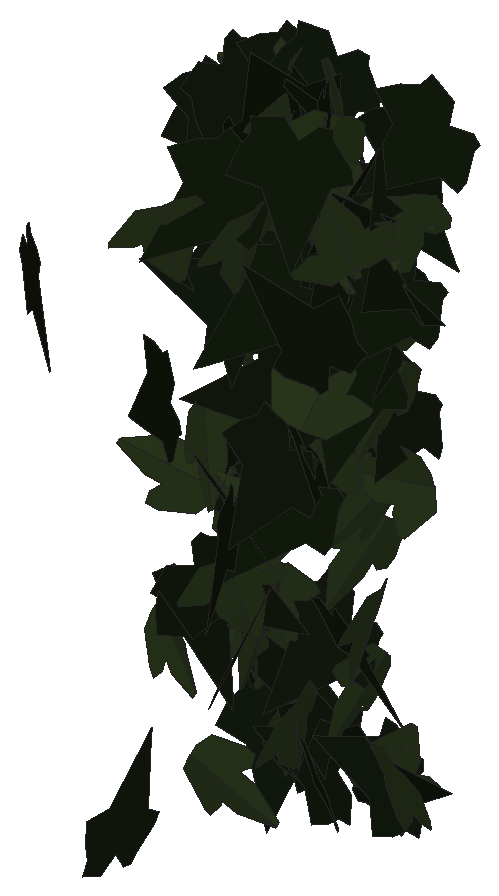
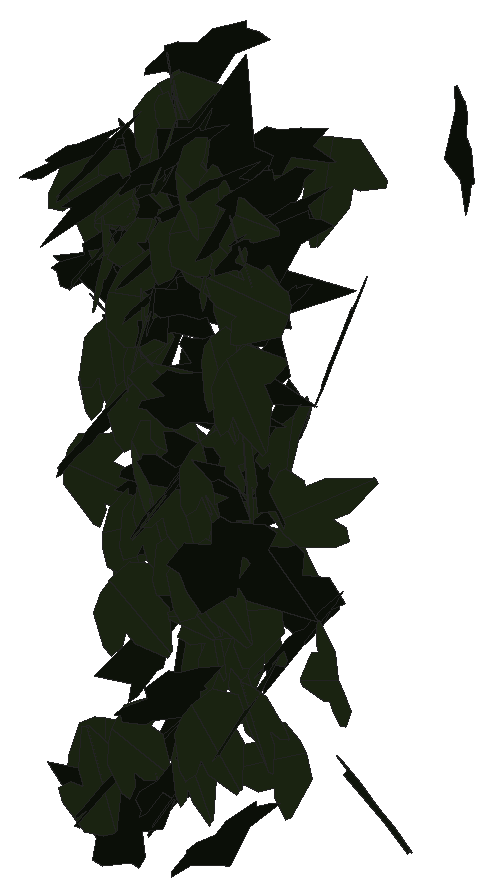
# SketchUp Ruby script. Lengths in inches.
U = 1.inch
M = Sketchup.active_model
def pt(a) = Geom::Point3d.new(a.map { |v| v * U })
def face(e, loops, mat)
  f = e.add_face(loops[0].map { |a| pt(a) })
  loops[1..].each { |l| e.add_face(l.map { |a| pt(a) }).erase! }
  f.material = f.back_material = mat if mat
  f
end
# faces: each face lists its corners as indices into pts; further lists are holes
def faces(e, pts, list, mat = nil) = list.each { |f| face(e, (f[0].is_a?(Array) ? f : [f]).map { |l| l.map { |i| pts[i] } }, mat) }
# xy, xz, yz: faces in a plane at the given z, y or x. An outline is a flat list of corners, or four numbers for a rectangle; further outlines are holes
def ring(l) = l.size == 4 ? [[l[0], l[1]], [l[2], l[1]], [l[2], l[3]], [l[0], l[3]]] : l.each_slice(2).to_a
def flat(e, list, mat, &to3) = list.each { |f| face(e, (f[0].is_a?(Array) ? f : [f]).map { |l| ring(l).map { |u, v| to3.(u, v) } }, mat) }
def xy(e, z, list, mat = nil) = flat(e, list, mat) { |x, y| [x, y, z] }
def xz(e, y, list, mat = nil) = flat(e, list, mat) { |x, z| [x, y, z] }
def yz(e, x, list, mat = nil) = flat(e, list, mat) { |y, z| [x, y, z] }
def lines(e, pts, list) = list.each { |a, b| e.add_line(pt(pts[a]), pt(pts[b])) }
# prism: a flat outline (further loops are holes) pulled along v
def prism(e, loops, v, mat = nil)
  f = face(e, loops, mat); d = Geom::Vector3d.new(v.map { |x| x * U })
  f.pushpull(f.normal.samedirection?(d) ? d.length : -d.length)
end
def box(e, o, s, mat = nil) = prism(e, [[o, [o[0] + s[0], o[1], o[2]], [o[0] + s[0], o[1] + s[1], o[2]], [o[0], o[1] + s[1], o[2]]]], [0, 0, s[2]], mat)
def at(x, y, z, deg = 0) = Geom::Transformation.translation(pt([x, y, z])) * Geom::Transformation.rotation(ORIGIN, Z_AXIS, deg.degrees)
def axes(o, x, y, z) = Geom::Transformation.new([*x, 0, *y, 0, *z, 0, *pt(o).to_a, 1])
def part(name) = M.definitions.add(name)
# library, detail: a bought-in or finely detailed component or shape, given as its bounding box
def library(name, o, s) = part(name).tap { |d| box(d.entities, o, s) }
def detail(e, o, s) = box(e.add_group.entities, o, s)
def put(e, d, t, mat = nil) = e.add_instance(d, t).tap { |i| i.material = mat if mat }
def group(e, t, mat = nil) = e.add_group.tap { |g| g.transformation = t; g.material = mat if mat }.entities
root = M.entities
M.materials.add("efeu1").color = [18, 25, 13]
M.materials.add("efeu2").color = [43, 57, 29]
c1 = part("ivyleaf_9")
p = [[1.54,2.16,1.25],[1.36,2.04,1.19],[-0.21,0.99,0.68],[-0.71,1.11,0.82],[-0.85,0.86,0.67],[-0.8,0.17,0.21],
  [-0.9,-0.01,0.1],[-0.67,-0.16,-0.02],[-0.08,-0.08,-0.05],[-0.03,-0.6,-0.4],[0.65,-0.88,-0.66],[0.83,-0.6,-0.49],
  [1.29,-0.42,-0.43],[1.8125,-0.07,-0.26],[1.21,0.44,0.15]]
faces(c1.entities,p,[[0,1,2,3,4,5,6,7,8,9,10,11,12,13,14]],"efeu1")
c2 = part("ivyleaf_10")
p = [[0,0.5,-0.03],[-0.0625,2.02,-0.43],[-0.19,2.01,-0.46],[-0.54,1.05,-0.29],[-0.52,0.625,-0.18],[-0.83,0.76,-0.28],
  [-1.16,0.64,-0.33],[-1.15,0.33,-0.24],[-0.77,-0.39,0.02],[-0.3,-0.51,0.16],[0.04,-0.48,0.23],[-0.02,2.01,-0.4375],
  [-0.06,2.01,-0.43],[0.04,-0.49,0.23],[0.67,-0.49,0.14],[1.38,0.36,-0.2],[1.375,0.51,-0.24],[0.81,0.65,-0.19],
  [0.62,0.59,-0.15],[0.6,1.09,-0.28],[0.5,1.23,-0.31]]
faces(c2.entities,p,[[0,1,2,3,4,5,6,7,8,9,10],[11,12,0,13,14,15,16,17,18,19,20]],"efeu2")
put(root,c1,axes([18.95,220.03,221.84],[-0.06149,0.00871,-0.49613],[0.49244,-0.0604,-0.06209],[-0.06101,-0.49626,-0.00115]))
put(root,c1,axes([21.28,220.7,216.89],[0.01146,0.41228,0.28266],[-0.00809,-0.28255,0.41243],[0.4998,-0.01403,0.0002]))
put(root,c1,axes([21.08,221.04,218.76],[-0.09206,0.04146,-0.4897],[0.42017,-0.25179,-0.10031],[-0.25492,-0.42998,0.01152]))
put(root,c1,axes([19.54,221.82,219.33],[-0.05656,-0.11309,0.48375],[-0.038,-0.48446,-0.1177],[0.49534,-0.05007,0.0462]))
put(root,c2,axes([19.75,221.52,221.93],[-0.3063,-0.38489,-0.08968],[0.04966,0.07509,-0.49183],[0.39207,-0.3102,-0.00777]))
put(root,c1,axes([19.13,221.41,213.57],[-0.39677,0.3007,-0.04643],[-0.03829,0.02635,0.49783],[0.30184,0.39861,0.00212]))
put(root,c1,axes([21.01,222.125,219.05],[-0.1345,-0.42098,0.23385],[-0.07876,-0.22031,-0.44188],[0.47509,-0.15571,-0.00705]))
put(root,c1,axes([21.24,222.05,223.16],[-0.14567,-0.4672,-0.10248],[0.04595,0.09296,-0.48913],[0.4761,-0.15192,0.01586]))
put(root,c1,axes([21.75,221.91,220.6],[0.03775,-0.03132,0.49759],[-0.42793,0.25402,0.04846],[-0.25583,-0.42953,-0.00762]))
put(root,c1,axes([20.21,222.29,222.21],[-0.36102,-0.2821,0.20022],[-0.15133,-0.13146,-0.45806],[0.31108,-0.39133,0.00954]))
put(root,c1,axes([19.95,222.14,218.31],[0.28926,-0.31716,0.25639],[0.17083,-0.19121,-0.42925],[0.37033,0.33593,-0.00226]))
put(root,c1,axes([21.22,222.25,218.6],[-0.45769,-0.19779,0.03745],[-0.03146,-0.02159,-0.49854],[0.19883,-0.45871,0.00731]))
put(root,c2,axes([20.4,222.16,221.77],[-0.03708,-0.49798,-0.02525],[0.00374,0.02504,-0.49936],[0.49861,-0.03722,0.00186]))
put(root,c2,axes([19.74,222.34,214.44],[-0.25172,0.04306,-0.42986],[0.42329,-0.07488,-0.25538],[-0.08636,-0.49248,0.00124]))
put(root,c1,axes([20.7,222.67,220.84],[-0.3923,-0.25823,0.17152],[-0.14312,-0.09453,-0.46966],[0.27499,-0.41759,0.00025]))
put(root,c2,axes([20.58,222.39,217.67],[0.28512,0.10776,0.39635],[-0.38992,-0.08063,0.30242],[0.12909,-0.48155,0.03806]))
put(root,c2,axes([19.62,222.43,218.85],[-0.02473,0.49027,-0.09498],[0.0056,-0.09481,-0.4909],[-0.49936,-0.02534,-0.0008]))
put(root,c2,axes([20.05,222.35,217.06],[-0.31514,-0.36391,-0.13513],[0.1015,0.09076,-0.4811],[0.37468,-0.33066,0.01667]))
put(root,c2,axes([21.27,222.23,219.68],[0.3131,0.30182,-0.24672],[0.1787,0.17012,0.43489],[0.34646,-0.36051,-0.00134]))
put(root,c1,axes([20.9375,222.76,214.58],[-0.04087,-0.12846,0.48148],[0.1398,-0.46666,-0.11264],[0.47832,0.12541,0.07406]))
put(root,c1,axes([20.24,222.52,220.51],[-0.19144,0.05148,0.45902],[-0.45168,0.08307,-0.1977],[-0.09662,-0.49036,0.0147]))
put(root,c2,axes([18.82,222.6,215.89],[0.20399,-0.07597,0.45013],[0.43929,-0.1014,-0.2162],[0.12413,0.48368,0.02538]))
put(root,c2,axes([20.9,222.39,215.49],[0.01818,-0.46905,-0.17223],[-0.00629,0.17211,-0.4694],[0.49963,0.01923,0.00035]))
put(root,c2,axes([19.33,222.65,217.89],[0.16218,0.21307,0.42225],[-0.26929,-0.32537,0.26762],[0.38882,-0.31422,0.00922]))
put(root,c1,axes([20.77,222.8,218.77],[0.0602,-0.28275,0.40796],[0.13901,-0.3849,-0.28728],[0.4765,0.14801,0.03227]))
put(root,c2,axes([21.52,222.67,221.52],[-0.27066,-0.37458,-0.19088],[-0.11407,-0.15307,0.46212],[-0.40464,0.2937,-0.0026]))
put(root,c1,axes([19.21,222.68,216.4375],[0.16806,-0.45698,-0.1137],[-0.02786,0.11087,-0.48676],[0.47008,0.16995,0.0118]))
put(root,c1,axes([20.69,222.78,219.46],[-0.12201,-0.12946,-0.46728],[-0.30996,-0.34972,0.17782],[-0.37288,0.33307,0.00508]))
put(root,c1,axes([19.52,222.4,216.91],[0.05267,-0.06948,-0.49234],[0.2039,0.45457,-0.04234],[0.45349,-0.19632,0.07622]))
put(root,c2,axes([20.85,222.83,222.8],[0.35587,-0.28701,0.20244],[0.15087,-0.13534,-0.45708],[0.31717,0.38641,-0.00972]))
put(root,c2,axes([20.99,222.9375,222.85],[-0.21171,-0.40186,0.20901],[-0.0478,-0.2096,-0.45142],[0.45044,-0.21112,0.05033]))
put(root,c1,axes([21.34,223,219.98],[-0.24726,-0.42789,-0.07595],[0.04304,0.06284,-0.49416],[0.43244,-0.25092,0.00576]))
put(root,c2,axes([20.03,222.98,216.39],[0.07766,-0.44952,0.20469],[0.08943,-0.19098,-0.45335],[0.48577,0.10703,0.05074]))
put(root,c1,axes([19.56,223.0625,220.56],[-0.00749,-0.49557,0.06598],[0.01257,-0.06615,-0.49544],[0.49979,-0.00577,0.01345]))
put(root,c1,axes([20.79,223.08,223],[-0.13957,-0.00862,-0.48005],[0.46526,-0.12587,-0.13302],[-0.11855,-0.48382,0.04315]))
put(root,c2,axes([20.89,222.79,221.92],[-0.45399,-0.07721,-0.19477],[0.19446,0.01777,-0.46029],[0.078,-0.49368,0.0139]))
put(root,c1,axes([19.85,222.55,218.34],[-0.03556,0.23017,0.44244],[-0.07409,0.43621,-0.23288],[-0.4932,-0.08212,0.00309]))
put(root,c1,axes([20.5,222.85,221.78],[0.31331,0.12325,-0.36965],[0.30034,0.22582,0.32985],[0.24826,-0.42873,0.06747]))
put(root,c1,axes([19.59,223.17,221.67],[0.03597,-0.10763,0.48695],[0.27192,-0.40502,-0.10961],[0.41805,0.27271,0.0294]))
put(root,c2,axes([19.59,223.14,215.91],[-0.16749,0.02967,0.47018],[0.43344,-0.18583,0.16613],[0.1846,0.46324,0.03653]))
put(root,c2,axes([21.49,223.09,216.81],[0.14228,-0.47469,0.06652],[0.02163,-0.06296,-0.49555],[0.47884,0.14389,0.00262]))
put(root,c1,axes([20.89,223.44,220.72],[-0.12363,-0.24737,0.41657],[0.03157,-0.43311,-0.24782],[0.48345,-0.03497,0.12271]))
put(root,c2,axes([19.9,223.11,218.37],[0.27699,-0.41584,-0.01875],[-0.00645,0.01824,-0.49963],[0.41622,0.27702,0.00474]))
put(root,c2,axes([20.54,223.02,217.93],[0.07563,0.49382,0.02051],[-0.03709,-0.01502,0.4984],[0.49285,-0.0769,0.03436]))
put(root,c1,axes([20.85,223.02,221.33],[0.03836,0.46327,0.18415],[-0.04447,-0.18078,0.46405],[0.49654,-0.05198,0.02734]))
put(root,c2,axes([20.64,223.18,218.49],[-0.44057,-0.13698,0.19271],[-0.16919,-0.10202,-0.45931],[0.16515,-0.46992,0.04354]))
put(root,c2,axes([21.03,223.52,219.45],[0.00981,-0.00523,-0.49988],[0.0028,-0.49996,0.00529],[-0.4999,-0.00291,-0.00978]))
put(root,c1,axes([20.02,223.34,222.41],[0.28118,0.17048,0.37666],[-0.32168,-0.19596,0.32882],[0.25974,-0.42724,-0.00053]))
put(root,c1,axes([21.68,223.53,220.88],[-0.3021,-0.36142,0.16767],[-0.10825,-0.12805,-0.47105],[0.38343,-0.3209,-0.00088]))
put(root,c2,axes([19.83,223.14,216.51],[-0.42148,-0.23056,-0.13854],[0.12943,0.05191,-0.48016],[0.2358,-0.44062,0.01592]))
put(root,c2,axes([20.05,223.41,222.6],[0.0207,-0.46395,0.18526],[0.00098,-0.18539,-0.46436],[0.49957,0.01958,-0.00677]))
put(root,c2,axes([20.1,223.38,217.93],[-0.26888,-0.35856,0.22167],[-0.1246,-0.18358,-0.44808],[0.40271,-0.2962,0.00936]))
put(root,c1,axes([19.89,222.96,218.04],[0.15051,-0.07106,-0.47149],[0.04563,0.49429,-0.05993],[0.47462,-0.02499,0.15528]))
put(root,c1,axes([19.04,223.63,222.23],[-0.18068,-0.42259,0.1969],[-0.00213,-0.21042,-0.45356],[0.46621,-0.16474,0.07423]))
put(root,c2,axes([20.84,223.15,221.1],[0.30938,0.05896,-0.38834],[0.38302,0.06431,0.3149],[0.08708,-0.49233,-0.00537]))
put(root,c2,axes([21.47,223.51,219.55],[-0.04659,-0.42566,0.25815],[0.02746,-0.26108,-0.42554],[0.49707,-0.02548,0.0477]))
put(root,c1,axes([21.47,223.71,220.99],[-0.11036,-0.27888,0.40006],[0.01783,-0.41221,-0.28243],[0.48734,-0.04807,0.10093]))
put(root,c1,axes([19.94,223.66,215.19],[0.05214,-0.45469,0.20135],[0.05052,-0.19657,-0.45696],[0.4947,0.06799,0.02545]))
put(root,c1,axes([20.32,223.66,222.64],[0.06846,-0.38152,0.31584],[0.16312,-0.28369,-0.37804],[0.46766,0.1548,0.08562]))
put(root,c1,axes([20.45,223.67,214.05],[0.12764,-0.47381,-0.09597],[0.05067,-0.0856,0.49001],[-0.48077,-0.13482,0.02616]))
put(root,c2,axes([19.82,223.7,221.53],[-0.02731,0.0731,-0.49387],[0.09266,-0.48528,-0.07695],[-0.49058,-0.09572,0.01296]))
put(root,c2,axes([21.11,222.99,221.79],[0.04015,-0.05389,-0.49546],[0.146,0.47653,-0.04],[0.47652,-0.14146,0.054]))
put(root,c2,axes([21.68,223.37,221.89],[-0.36178,-0.34494,0.01121],[-0.00364,-0.01242,-0.49983],[0.34511,-0.36174,0.00648]))
put(root,c1,axes([21.5,223.39,220.1],[-0.43472,0.23341,0.08087],[-0.07738,0.02677,-0.49325],[-0.23459,-0.44136,0.01285]))
put(root,c2,axes([21.24,223.375,221.75],[0.41043,0.27487,0.07742],[0.05738,0.05341,-0.49382],[-0.27974,0.41424,0.0123]))
put(root,c1,axes([20.65,223.49,216.13],[0.36028,-0.33407,0.09271],[0.06831,-0.06268,-0.49133],[0.3399,0.3667,0.00047]))
put(root,c1,axes([20.52,223.78,220.78],[-0.02671,-0.05187,0.49658],[-0.05066,-0.49445,-0.05437],[0.49671,-0.05322,0.02116]))
put(root,c1,axes([20.71,223.46,220.62],[0.07605,-0.05008,0.49164],[-0.44657,0.20606,0.09007],[-0.21163,-0.4528,-0.01338]))
put(root,c1,axes([18.97,223.68,222.1],[-0.1139,-0.48374,-0.05498],[0.01336,0.05333,-0.49697],[0.48667,-0.11468,0.00078]))
put(root,c2,axes([19.62,223.42,221.39],[-0.49089,-0.06914,0.06518],[-0.06407,-0.01243,-0.49572],[0.07016,-0.49504,0.00335]))
put(root,c2,axes([20.13,223.62,214.95],[0.08399,-0.47866,0.11761],[0.04065,-0.11217,-0.48556],[0.49122,0.09112,0.02007]))
put(root,c2,axes([20.69,223.8,220.5],[-0.0273,0.13189,-0.48152],[0.146,-0.45905,-0.13401],[-0.47743,-0.14792,-0.01345]))
put(root,c1,axes([20.84,223.49,220.68],[0.23661,-0.03865,-0.43877],[0.39592,0.23694,0.19263],[0.19303,-0.4386,0.14273]))
put(root,c2,axes([19.45,223.38,218.96],[0.26258,-0.3479,-0.24499],[-0.08,0.24238,-0.42994],[0.41791,0.26499,0.07162]))
put(root,c2,axes([19.51,223.6,222.28],[0.28009,-0.41328,0.02734],[0.01294,-0.02426,-0.49924],[0.41398,0.28038,-0.00289]))
put(root,c1,axes([20.08,223.81,221.1],[-0.4031,-0.28686,0.07228],[-0.05454,-0.04801,-0.49469],[0.29075,-0.4067,0.00742]))
put(root,c2,axes([21.61,223.41,214.47],[-0.43747,0.14213,0.196],[-0.18467,0.06587,-0.45996],[-0.15657,-0.47482,-0.00514]))
put(root,c2,axes([20.76,223.71,219.43],[-0.27377,-0.2266,0.35171],[-0.27622,-0.2178,-0.35534],[0.31425,-0.38886,-0.00593]))
put(root,c2,axes([19.8,223.73,218.42],[0.34726,-0.17106,0.31646],[0.29294,-0.12082,-0.38676],[0.20878,0.45403,0.01631]))
put(root,c1,axes([20.41,223.94,221.02],[-0.06206,-0.43845,0.23218],[-0.00818,-0.23305,-0.44229],[0.49607,-0.0587,0.02175]))
put(root,c2,axes([20.46,223.64,223.02],[-0.25923,0.36942,-0.21524],[0.1286,-0.17269,-0.45127],[-0.40775,-0.28932,-0.00548]))
put(root,c1,axes([21.37,223.99,222.33],[-0.09235,-0.38959,0.29949],[-0.01546,-0.30228,-0.39798],[0.49115,-0.08276,0.04378]))
put(root,c2,axes([20.87,223.98,217.73],[0.00538,-0.11598,0.48633],[0.13569,-0.46777,-0.11306],[0.48121,0.13319,0.02645]))
put(root,c1,axes([19.15,223.95,215.79],[0.06538,-0.40411,0.28709],[0.03879,-0.28452,-0.40932],[0.49419,0.0758,-0.00585]))
put(root,c2,axes([19.71,223.79,218.98],[-0.10414,-0.45803,0.17137],[0.02485,-0.17994,-0.46584],[0.4884,-0.08851,0.06024]))
put(root,c1,axes([20.4,223.62,214.3],[-0.2202,-0.3942,0.21476],[0.10369,0.18807,0.45153],[-0.43676,0.24339,-0.00108]))
put(root,c2,axes([21.23,223.68,219.97],[-0.09809,-0.49025,0.00596],[-0.00143,-0.00579,-0.49996],[0.49028,-0.0981,-0.00026]))
put(root,c1,axes([20.47,223.63,221.4375],[0.19491,-0.40698,-0.21536],[-0.04499,0.2159,-0.44873],[0.45824,0.1943,0.04754]))
put(root,c2,axes([19.15,223.72,216.03],[0.46452,-0.18483,-0.0079],[-0.00778,0.00182,-0.49994],[0.18483,0.46458,-0.00119]))
put(root,c1,axes([20.21,223.98,218.46],[0.04204,-0.45539,0.20212],[0.00071,-0.20278,-0.45703],[0.49823,0.03871,-0.0164]))
put(root,c1,axes([19.02,223.51,222.74],[0.17421,-0.2902,-0.36802],[-0.05022,0.3788,-0.32247],[0.46597,0.14932,0.10283]))
put(root,c1,axes([20.06,223.49,218.75],[0.30761,-0.23956,-0.31303],[-0.1476,0.29817,-0.37324],[0.3655,0.32203,0.11272]))
put(root,c2,axes([19.01,223.6,221.16],[0.15781,-0.03124,-0.47341],[0.47355,0.04101,0.15514],[0.02914,-0.49733,0.04254]))
put(root,c2,axes([21.59,223.69,218.17],[0.0822,0.01172,-0.49306],[-0.48607,0.08657,-0.07897],[0.08352,0.49231,0.02563]))
put(root,c2,axes([21.11,223.98,221.31],[-0.0967,0.22114,-0.43789],[0.10608,-0.42633,-0.23872],[-0.47895,-0.13907,0.03554]))
put(root,c1,axes([21.14,223.64,222.1],[0.19432,-0.37072,-0.2735],[0.03384,0.30752,-0.39279],[0.45945,0.13414,0.14461]))
put(root,c1,axes([20.33,224.07,215.76],[-0.27427,-0.36734,0.19959],[-0.11329,-0.16448,-0.45838],[0.40242,-0.29667,0.00699]))
put(root,c1,axes([21.23,224.01,214.01],[0.04979,-0.48589,-0.10691],[0.01423,-0.10601,0.48843],[-0.49731,-0.05168,0.00327]))
put(root,c2,axes([19.23,223.87,220.25],[-0.02706,-0.47942,0.13936],[-0.00662,-0.13921,-0.48018],[0.49922,-0.02783,0.00118]))
put(root,c2,axes([20.5,223.83,218.09],[-0.14391,-0.4681,0.10087],[-0.0166,-0.10039,-0.48954],[0.47855,-0.14425,0.01335]))
put(root,c2,axes([19.18,223.5625,217.09],[-0.07007,-0.04406,-0.4931],[0.46364,0.16877,-0.08096],[0.17358,-0.46859,0.0172]))
put(root,c2,axes([19.69,224.15,222.14],[-0.08935,-0.06229,0.48799],[0.00383,-0.49605,-0.06262],[0.49194,-0.00745,0.08913]))
put(root,c2,axes([20.65,224.14,220.97],[-0.03235,-0.21232,0.45152],[0.09261,-0.44716,-0.20364],[0.49028,0.07046,0.06826]))
put(root,c2,axes([19.94,223.97,222.01],[-0.20325,-0.39877,0.22287],[-0.07211,-0.21286,-0.44664],[0.4511,-0.2137,0.02901]))
put(root,c1,axes([19.37,224.0625,214.29],[-0.05131,-0.49528,0.04546],[0.0047,-0.04618,-0.49784],[0.49734,-0.05066,0.00939]))
put(root,c1,axes([20.05,224.07,219.83],[-0.39604,-0.17451,0.2504],[-0.23143,-0.09572,-0.43276],[0.19897,-0.45868,-0.00496]))
put(root,c2,axes([19.95,223.81,217.71],[-0.42634,-0.1126,0.23571],[-0.22404,-0.07437,-0.44077],[0.13432,-0.48145,0.01296]))
put(root,c1,axes([19.66,224.2,222.62],[-0.24828,-0.36196,0.23946],[-0.03609,-0.2577,-0.42695],[0.4325,-0.22929,0.10183]))
put(root,c1,axes([19.69,223.76,218.74],[0.08469,-0.08258,-0.48581],[0.38211,0.32226,0.01183],[0.31116,-0.37327,0.11769]))
put(root,c1,axes([20.13,224.12,222.96],[-0.09847,-0.48334,0.08178],[0.0073,-0.08485,-0.49269],[0.49015,-0.09584,0.02377]))
put(root,c1,axes([19.42,224.02,218.03],[0.02766,0.03632,-0.49791],[-0.22925,-0.44206,-0.04498],[-0.44349,0.23078,-0.0078]))
put(root,c2,axes([19.6,224.03,215.66],[-0.0805,-0.44874,0.20531],[-0.03047,-0.20311,-0.45587],[0.49254,-0.08591,0.00535]))
put(root,c2,axes([20.16,223.86,218.54],[-0.42429,-0.16613,0.20586],[-0.19338,-0.07073,-0.45563],[0.18051,-0.46626,-0.00423]))
put(root,c2,axes([20.48,224.04,218.875],[0.20094,-0.41231,0.19906],[0.09882,-0.17321,-0.45851],[0.44705,0.22361,0.01188]))
put(root,c1,axes([20.03,223.98,218.83],[-0.2758,-0.33308,-0.25099],[0.18915,0.16827,-0.43117],[0.37169,-0.33278,0.03319]))
put(root,c1,axes([21.18,224.24,218.95],[-0.05556,-0.40273,0.29107],[-0.02649,-0.29007,-0.4064],[0.4962,-0.06058,0.0109]))
put(root,c2,axes([20.8125,223.63,221.43],[-0.09074,0.42426,0.24853],[-0.1388,0.22035,-0.42683],[-0.4717,-0.14645,0.07779]))
put(root,c2,axes([19.73,224.15,222.81],[0.17259,-0.32329,0.34014],[0.17243,-0.29337,-0.36634],[0.43644,0.24376,0.01023]))
put(root,c2,axes([19.72,223.94,217.6],[-0.34451,-0.0842,0.35245],[-0.32728,-0.13647,-0.35251],[0.15556,-0.47359,0.03892]))
put(root,c2,axes([20.6,224.18,215.17],[0.04927,-0.35545,0.34818],[0.06413,-0.34242,-0.35865],[0.49342,0.08,0.01185]))
put(root,c2,axes([19.51,223.84,222.34],[0.11557,0.04669,0.48421],[-0.48544,-0.02109,0.1179],[0.03144,-0.49737,0.04046]))
put(root,c2,axes([20.68,224.14,217],[-0.09773,-0.39718,0.28757],[-0.04421,-0.28489,-0.40851],[0.48836,-0.10528,0.02057]))
put(root,c1,axes([20.61,223.96,213.91],[0.15718,-0.09625,0.46479],[0.40015,-0.23646,-0.18429],[0.25529,0.42991,0.0027]))
put(root,c2,axes([21.03,223.93,213.98],[-0.42704,-0.2093,0.15438],[0.14312,0.05869,0.47547],[-0.21716,0.45028,0.00979]))
put(root,c2,axes([19.41,223.99,220.5],[0.09722,-0.4899,0.02337],[-0.00077,-0.02397,-0.49942],[0.49046,0.09707,-0.00542]))
put(root,c1,axes([21.56,224.3125,222.51],[-0.29781,-0.29761,0.26969],[-0.07095,-0.29148,-0.4],[0.39532,-0.27652,0.13138]))
